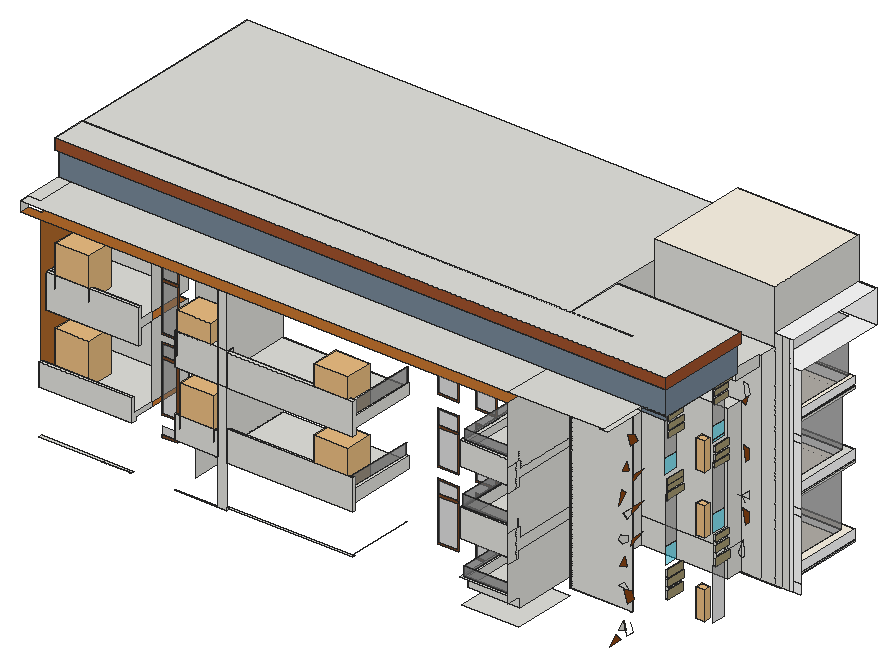
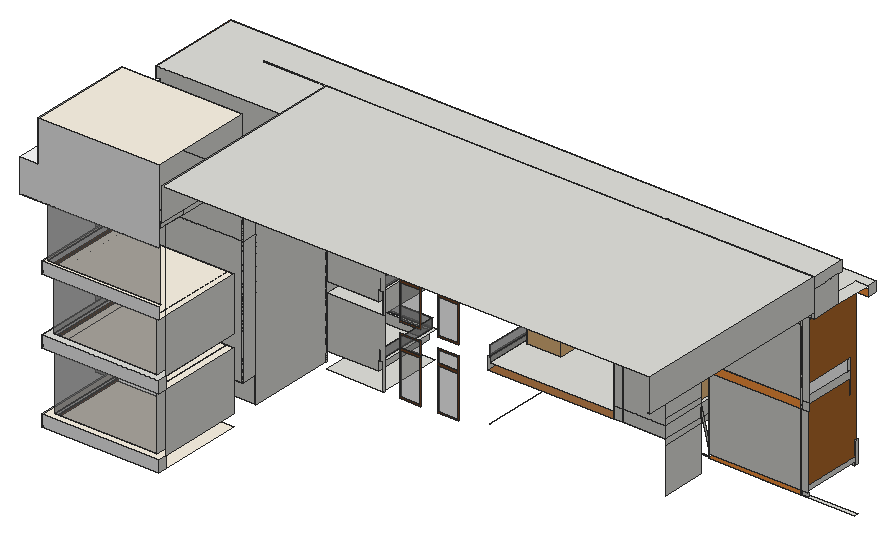
# SketchUp Ruby script. Lengths in inches.
U = 1.inch
M = Sketchup.active_model
def pt(a) = Geom::Point3d.new(a.map { |v| v * U })
def face(e, loops, mat)
  f = e.add_face(loops[0].map { |a| pt(a) })
  loops[1..].each { |l| e.add_face(l.map { |a| pt(a) }).erase! }
  f.material = f.back_material = mat if mat
  f
end
# faces: each face lists its corners as indices into pts; further lists are holes
def faces(e, pts, list, mat = nil) = list.each { |f| face(e, (f[0].is_a?(Array) ? f : [f]).map { |l| l.map { |i| pts[i] } }, mat) }
# xy, xz, yz: faces in a plane at the given z, y or x. An outline is a flat list of corners, or four numbers for a rectangle; further outlines are holes
def ring(l) = l.size == 4 ? [[l[0], l[1]], [l[2], l[1]], [l[2], l[3]], [l[0], l[3]]] : l.each_slice(2).to_a
def flat(e, list, mat, &to3) = list.each { |f| face(e, (f[0].is_a?(Array) ? f : [f]).map { |l| ring(l).map { |u, v| to3.(u, v) } }, mat) }
def xy(e, z, list, mat = nil) = flat(e, list, mat) { |x, y| [x, y, z] }
def xz(e, y, list, mat = nil) = flat(e, list, mat) { |x, z| [x, y, z] }
def yz(e, x, list, mat = nil) = flat(e, list, mat) { |y, z| [x, y, z] }
def lines(e, pts, list) = list.each { |a, b| e.add_line(pt(pts[a]), pt(pts[b])) }
# prism: a flat outline (further loops are holes) pulled along v
def prism(e, loops, v, mat = nil)
  f = face(e, loops, mat); d = Geom::Vector3d.new(v.map { |x| x * U })
  f.pushpull(f.normal.samedirection?(d) ? d.length : -d.length)
end
def box(e, o, s, mat = nil) = prism(e, [[o, [o[0] + s[0], o[1], o[2]], [o[0] + s[0], o[1] + s[1], o[2]], [o[0], o[1] + s[1], o[2]]]], [0, 0, s[2]], mat)
def at(x, y, z, deg = 0) = Geom::Transformation.translation(pt([x, y, z])) * Geom::Transformation.rotation(ORIGIN, Z_AXIS, deg.degrees)
def axes(o, x, y, z) = Geom::Transformation.new([*x, 0, *y, 0, *z, 0, *pt(o).to_a, 1])
def part(name) = M.definitions.add(name)
# library, detail: a bought-in or finely detailed component or shape, given as its bounding box
def library(name, o, s) = part(name).tap { |d| box(d.entities, o, s) }
def detail(e, o, s) = box(e.add_group.entities, o, s)
def put(e, d, t, mat = nil) = e.add_instance(d, t).tap { |i| i.material = mat if mat }
def group(e, t, mat = nil) = e.add_group.tap { |g| g.transformation = t; g.material = mat if mat }.entities
root = M.entities
M.materials.add("[0030_OldLace]").color = [253, 245, 230]
M.materials.add("[0042_Sienna]").color = [160, 82, 45]
M.materials.add("[0043_SaddleBrown]").color = [139, 69, 19]
M.materials.add("[0110_LightSlateGray]").color = [119, 136, 153]
M.materials.add("[0128_White]").color = [255, 255, 255]
M.materials.add("[Translucent Glass Gray]").color = [128, 128, 128]
M.materials["[Translucent Glass Gray]"].alpha = 0.5
M.materials.add("[Translucent Glass Tinted]").color = [8, 201, 241]
M.materials["[Translucent Glass Tinted]"].alpha = 0.48
M.materials.add("[Wood Bamboo]").color = [177, 105, 43]
M.materials.add("[Wood Floor]").color = [155, 105, 61]
M.materials.add("[Wood Lumber ButtJoined]").color = [164, 152, 112]
M.materials.add("[Wood Veneer 01]").color = [120, 70, 37]
c1 = library("WALL+LIGHT+69",[4.19,4.05,-9.67],[4.61,5.7,18.91])
c2 = library("Plant+(3)",[-15.5,2.64,0],[117.71,96.38,184.75])
xy(root,304.04,[[1381.11,725.91,1632.4375,929.16]],"[0030_OldLace]")
xy(root,305.16,[[1631,725.91,1632.4375,929.16]])
xy(root,306.29,[[1631,725.91,1632.4375,929.16]])
xy(root,307.875,[[1256.11,342.41,1378.67,480.63]])
xy(root,307.92,[[1631,725.91,1632.4375,929.16]])
xy(root,309.05,[[1631,725.91,1632.4375,929.16]])
xy(root,320.91,[[648.14,329.32,760.05,331.76]])
xy(root,321.16,[[356.17,329.32,555.3,336.26]])
xy(root,322.75,[[1378.67,480.63,1512.23,481.99]])
xy(root,326.04,[[760.05,329.32,1031.24,336.23],[1025.87,336.23,1026.95,480.63]])
xy(root,328.75,[[1381.11,725.91,1381.11,929.16,1632.4375,929.16,1632.4375,725.91,1616.3,725.91,1616.3,913.03,1397.24,913.03,1397.24,725.91]],"[0030_OldLace]")
xy(root,344.1875,[[1266.15,344.87,1378.67,480.63]])
xy(root,364.5625,[[1256.11,335.28,1378.67,335.28,1378.67,340.07,1261.86,340.07,1261.86,480.63,1256.11,480.63],[1263.19,341.7,1378.67,341.7,1378.67,344.87,1266.15,344.87,1266.15,480.63,1263.19,480.63]])
xy(root,379.5625,[[1378.67,669.54,1381.11,703.91],[1381.11,669.54,1567.08,703.91]])
xy(root,385.9375,[[1261.86,340.07,1378.67,340.07,1378.67,341.7,1263.19,341.7,1263.19,480.63,1261.86,480.63]])
xy(root,411.86,[[1627.32,427.98,1631.63,468.55]])
xy(root,413.45,[[760.05,329.32,1031.24,333.68]])
xy(root,417.33,[[648.14,329.32,740.81,330.51]])
xy(root,417.38,[[760.05,333.68,1031.24,334.64]])
xy(root,417.48,[[356.17,329.32,356.17,335.25,540.9,335.25,540.9,341.375,555.3,341.375,555.3,329.32]])
xy(root,417.71,[[1625.18,558.89,1628.93,596.95]])
xy(root,425.41,[[341.11,480.02,356.17,480.63]])
xy(root,425.41,[[356.17,335.25,356.17,480.63,555.3,480.63,555.3,341.375,540.9,341.375,540.9,335.25]],"[Wood Bamboo]")
xy(root,429.39,[[1627.32,427.98,1631.63,468.55]])
xy(root,429.57,[[648.14,330.51,740.81,480.63],[760.05,334.64,1031.24,480.63]],"[Wood Floor]")
xy(root,433.35,[[1625.18,558.89,1628.93,596.95]])
xy(root,434.15,[[356.17,335.79,555.3,480.63],[341.11,480.01,356.17,480.63]])
xy(root,435.78,[[1627.32,427.98,1631.63,470.67]])
xy(root,439.59,[[1256.11,335.28,1378.67,341.89]])
xy(root,443.1,[[1625.18,558.89,1628.93,594.7]])
xy(root,444.84,[[760.05,333.68,1024.58,480.63]])
xy(root,450.52,[[1627.32,427.98,1631.63,470.67]])
xy(root,454.4,[[1627.32,427.98,1631.63,467.8]])
xy(root,455.53,[[648.14,333.49,740.81,480.63],[1026.48,333.68,1031.24,480.63],[1256.11,341.89,1378.67,480.63]])
xy(root,456.06,[[1397.24,725.91,1616.3,913.03]])
xy(root,456.48,[[1381.11,725.91,1632.4375,929.16]],"[0030_OldLace]")
xy(root,457.13,[[1625.18,558.89,1628.93,594.7]])
xy(root,458.99,[[1630.3125,725.91,1632.4375,929.16]])
xy(root,460.73,[[1630.3125,725.91,1632.4375,929.16]])
xy(root,462.54,[[1630.3125,725.91,1632.4375,929.16]])
xy(root,464.25,[[1630.3125,725.91,1632.4375,929.16]])
xy(root,464.84,[[1625.18,558.89,1628.93,594.2]])
xy(root,466.46,[[356.17,329.32,555.3,335.79]])
xy(root,467.97,[[648.14,329.32,740.81,333.49]])
xy(root,468.47,[[1627.32,427.98,1631.63,467.8]])
xy(root,476.71,[[1625.18,558.89,1628.93,594.2]])
xy(root,478.58,[[1265.15,344.3125,1378.67,480.63]])
xy(root,478.66,[[760.05,329.32,1031.24,333.68],[1024.58,333.68,1026.48,480.63]])
xy(root,482.34,[[1381.11,725.91,1381.11,929.16,1632.4375,929.16,1632.4375,725.91,1617.91,725.91,1617.91,914.63,1395.63,914.63,1395.63,728.87,1583.5,728.87,1583.5,725.91]])
xy(root,500.08,[[1256.11,335.28,1378.67,335.28,1378.67,339.79,1260.73,339.79,1260.73,480.63,1256.11,480.63],[1261.13,340.29,1378.67,340.29,1378.67,344.3125,1265.15,344.3125,1265.15,480.63,1261.13,480.63]])
xy(root,523.64,[[1260.73,339.79,1378.67,339.79,1378.67,340.29,1261.13,340.29,1261.13,480.63,1260.73,480.63]])
xy(root,558.06,[[648.14,329.32,760.05,347.69],[760.05,329.32,1031.24,337.57]])
xy(root,558.97,[[356.17,347.69,555.3,353.19]])
xy(root,572.25,[[648.14,331.57,740.81,347.69]])
xy(root,572.25,[[760.05,337.57,1031.24,480.63],[648.14,347.69,740.81,480.63]],"[Wood Floor]")
xy(root,578.13,[[1256.11,335.28,1378.67,342.54]])
xy(root,588.63,[[760.05,337.57,1026.8,480.63]])
xy(root,590.28,[[341.11,479.78,356.17,480.63]])
xy(root,590.28,[[356.17,353.19,555.3,480.63]],"[Wood Bamboo]")
xy(root,595.76,[[648.14,331.57,740.81,480.63],[1028.375,337.57,1031.24,480.63],[1256.11,342.54,1378.67,480.63]])
xy(root,597.41,[[1583.5,725.91,1583.5,728.87,1395.63,728.87,1395.63,914.63,1617.91,914.63,1617.91,725.91]])
xy(root,598.78,[[1381.11,725.91,1632.4375,929.16]],"[0030_OldLace]")
xy(root,602.32,[[1630.1875,725.91,1632.4375,929.16]])
xy(root,604.08,[[1630.1875,725.91,1632.4375,929.16]])
xy(root,605.18,[[1629.07,427.98,1631.5,469.55]])
xy(root,605.42,[[1630.3125,725.91,1632.4375,929.16]])
xy(root,606.8,[[1623.49,558.89,1627.24,595.51]])
xy(root,607.68,[[1630.3125,725.91,1632.4375,929.16]])
xy(root,607.98,[[356.17,355.38,555.3,479.76]])
xy(root,611.84,[[1268.92,348.09,1378.67,480.63]])
xy(root,616.24,[[1623.49,558.89,1627.24,595.51]])
xy(root,616.93,[[1629.07,427.98,1631.5,469.55]])
xy(root,620.41,[[1624.9,558.89,1628.78,594.07]])
xy(root,621.03,[[1629.07,427.98,1631.5,468.05]])
xy(root,624.41,[[1625.07,725.91,1625.07,922.47,1381.11,922.47,1381.11,929.16,1632.4375,929.16,1632.4375,725.91]],"[0030_OldLace]")
xy(root,625.94,[[760.05,329.32,1031.24,337.57],[1026.8,337.57,1028.375,480.63]])
xy(root,628.4,[[1256.11,335.28,1378.67,335.28,1378.67,341.58,1262.51,341.58,1262.51,480.63,1256.11,480.63],[1263.04,342.52,1378.67,342.52,1378.67,348.09,1268.92,348.09,1268.92,480.63,1263.04,480.63]])
xy(root,629.13,[[648.14,329.32,760.05,347.69]])
xy(root,630.5,[[1629.07,427.98,1631.5,468.05]])
xy(root,630.91,[[1624.9,558.89,1628.78,594.07]])
xy(root,631.73,[[356.17,347.69,555.3,355.38]])
xy(root,633.43,[[1629.07,427.98,1631.5,467.67]])
xy(root,636.65,[[1624.78,558.89,1628.78,594.34]])
xy(root,643.95,[[1629.07,427.98,1631.5,467.67]])
xy(root,649.25,[[1624.78,558.89,1628.78,594.34]])
xy(root,649.4,[[1262.51,341.58,1263.04,480.63],[1263.04,341.58,1378.67,342.52]])
xy(root,651.9375,[[1378.67,669.54,1567.08,703.91]])
xy(root,723.3125,[[1630.2,427.98,1632.07,468.05]])
xy(root,728.9,[[1624.7,558.89,1626.82,594.34]])
xy(root,735.53,[[1630.2,427.98,1632.07,468.05]])
xy(root,738.98,[[1381.11,922.47,1583.5,929.53]])
xy(root,738.98,[[1625.07,725.91,1678.36,725.91,1678.36,929.53,1583.5,929.53,1583.5,922.47,1625.07,922.47]],"[0128_White]")
xy(root,739.45,[[1630.2,427.98,1632.07,469.17]])
xy(root,740.75,[[1624.7,558.89,1626.82,594.34]])
xy(root,745.11,[[1624.7,558.89,1626.82,593.95]])
xy(root,747.5625,[[740.81,329.32,760.05,480.63]])
xy(root,750.7,[[1630.2,427.98,1632.07,469.17]])
xy(root,751.9375,[[555.3,384.82,648.14,479.76]])
xy(root,752.13,[[328.44,313.35,328.44,334.16,356.17,334.16,356.17,384.82,648.14,384.82,648.14,480.63,1378.67,480.63,1378.67,313.35],[356.17,384.82,648.14,415.98],[356.17,415.98,648.14,479.76]],"[Wood Bamboo]")
xy(root,755.19,[[1624.7,558.89,1626.82,593.95]])
xy(root,757.41,[[1618,606,1635.25,666.21]])
xy(root,757.6,[[1630.2,427.98,1632.07,467.07]])
xy(root,758.84,[[1624.7,558.89,1626.82,606]])
xy(root,764,[[1566.87,325.97,1584.12,415.98]])
xy(root,767.17,[[1624.7,558.89,1626.82,606]])
xy(root,768.01,[[1630.2,427.98,1632.07,467.07]])
xy(root,770.68,[[1621.75,427.98,1636.25,467.07],[1632.37,467.07,1636.25,558.89],[1621.75,558.89,1636.25,594.34]])
xy(root,774.125,[[328.44,313.35,1378.67,313.35,1379.01,415.98,356.17,415.98,356.17,334.16,328.44,334.16],[1378.67,313.35,1584.12,313.35,1584.12,415.98,1379.01,415.98],[328.44,334.16,356.17,415.98],[328.44,479.76,341.11,480.63]])
xy(root,781.4375,[[1378.67,606,1635.25,606,1635.25,666.21,1639.62,666.21,1639.62,703.91,1378.67,703.91]])
xy(root,784.875,[[341.11,479.76,356.17,480.63],[328.44,480.63,334.36,922.03],[334.36,480.63,341.11,863.91],[1378.67,480.63,1381.11,480.63,1381.11,703.91,1380.23,703.91,1380.59,789.03,1380.91,863.91,1380.91,922.03,1378.67,922.03]])
xy(root,808.62,[[1639.62,703.91,1678.36,929.53]],"[0128_White]")
xy(root,831.95,[[328.44,405.29,328.44,415.98,1636.25,415.98,1636.25,606,1644.87,606,1644.87,405.29]],"[Wood Bamboo]")
xy(root,855,[[328.44,405.29,1644.87,405.29,1644.87,606,1378.67,606,1378.67,481.99,1512.23,481.99,1512.23,480.63,648.14,480.63,648.14,479.76,328.44,479.76],[356.17,479.76,648.14,480.63],[328.44,480.63,1378.67,922.03]])
xy(root,897.8125,[[1381.11,703.91,1639.62,929.53]],"[0030_OldLace]")
xz(root,329.32,[[740.81,320.91,760.05,558.06],[555.3,321.06,555.3,321.16,490.96,321.16],[760.05,413.45,1031.24,478.66],[648.14,417.33,740.81,467.97],[356.17,417.48,555.3,466.46],
  [648.14,558.06,740.81,629.13],[740.81,558.06,760.05,629.13],[760.05,558.06,1031.24,625.94],[740.81,629.13,760.05,747.5625]])
xz(root,330.51,[[648.14,417.33,740.81,429.57]])
xz(root,331.57,[[648.14,572.25,740.81,595.76]])
xz(root,333.49,[[648.14,455.53,740.81,467.97]])
xz(root,333.68,[[760.05,413.45,1031.24,417.38],[760.05,444.84,1024.58,478.66],[1026.48,455.53,1031.24,478.66]])
xz(root,334.64,[[760.05,417.38,1031.24,429.57]])
xz(root,335.25,[[356.17,417.48,540.9,425.41]])
xz(root,335.28,[[1256.11,439.59,1378.67,500.08],[1256.11,578.13,1378.67,628.4]])
xz(root,335.79,[[356.17,434.15,555.3,466.46]])
xz(root,337.57,[[760.05,558.06,1031.24,572.25],[760.05,588.63,1026.8,625.94],[1028.375,595.76,1031.24,625.94]])
xz(root,339.79,[[1260.73,500.08,1378.67,523.64]],"[Translucent Glass Gray]")
xz(root,340.07,[[1261.86,364.5625,1378.67,385.9375]],"[Translucent Glass Gray]")
xz(root,340.29,[[1261.13,500.08,1378.67,523.64]],"[Translucent Glass Gray]")
xz(root,341.375,[[540.9,417.48,555.3,425.41]])
xz(root,341.58,[[1262.51,628.4,1263.04,649.4]])
xz(root,341.58,[[1263.04,628.4,1378.67,649.4]],"[Translucent Glass Gray]")
xz(root,341.7,[[1263.19,364.5625,1378.67,385.9375]],"[Translucent Glass Gray]")
xz(root,341.89,[[1256.11,439.59,1378.67,455.53]])
xz(root,342.52,[[1263.04,628.4,1378.67,649.4]],"[Translucent Glass Gray]")
xz(root,342.54,[[1256.11,578.13,1378.67,595.76]])
xz(root,344.3125,[[1265.15,478.58,1378.67,500.08]])
xz(root,344.87,[[1266.15,344.1875,1378.67,364.5625]])
xz(root,347.69,[[648.14,558.06,740.81,572.25],[356.17,558.97,555.3,631.73],[648.14,595.76,736.24,629.13]])
xz(root,348.09,[[1268.92,611.84,1378.67,628.4]])
xz(root,353.19,[[356.17,558.97,555.3,590.28]])
xz(root,355.38,[[356.17,607.98,555.3,631.73]])
xz(root,384.82,[[578.02,378.89,609.9,395.73],[578.83,420.27,609.08,525.18],[578.83,530.5625,609.08,555.125],[578.25,574.6,609.66,673.69],[578.25,679.55,609.66,704.65]],"[Translucent Glass Gray]")
xz(root,384.82,[[575.9,373.61,578.02,378.89],[578.02,373.61,609.9,378.89],[[575.9,417.33,612.02,558.06],[578.83,420.27,609.08,555.125]],[578.83,525.18,609.08,530.5625],[575.9,572.25,612.02,572.25,612.02,707,575.9,707,575.9,679.55,578.25,679.55,578.25,704.65,609.66,704.65,609.66,574.6,578.25,574.6,578.25,673.69,575.9,673.69],
  [575.9,673.69,578.25,679.55],[578.25,673.69,609.66,679.55]],"[Wood Veneer 01]")
xz(root,405.29,[[328.44,831.95,1644.87,855]],"[0042_Sienna]")
xz(root,415.98,[[1584.12,764,1636.25,770.68],[1584.12,770.68,1636.25,774.125],[328.44,774.125,1636.25,831.95]],"[0110_LightSlateGray]")
xz(root,427.98,[[1627.32,429.39,1631.63,435.78],[1627.32,450.52,1631.63,454.4],[1629.07,602.14,1631.5,605.18],[1629.07,616.93,1631.5,618.39],[1629.07,618.39,1631.5,621.03],
  [1629.07,630.5,1631.5,633.43],[1630.2,735.53,1632.07,739.45],[1630.2,739.45,1632.07,750.7],[1630.2,750.7,1632.07,757.6],[1630.2,768.01,1632.07,769.27]])
xz(root,467.07,[[1630.2,757.6,1632.07,768.01],[1632.07,766.85,1632.37,768.01]])
xz(root,467.67,[[1629.07,633.43,1631.5,643.95]])
xz(root,467.8,[[1627.32,454.4,1631.63,468.47]])
xz(root,468.05,[[1629.07,621.03,1631.5,630.5],[1630.2,723.3125,1632.07,735.53]])
xz(root,468.55,[[1627.32,411.86,1631.63,429.39]])
xz(root,469.17,[[1630.2,739.45,1632.07,750.7]])
xz(root,469.55,[[1629.07,605.18,1631.5,616.93]])
xz(root,470.67,[[1627.32,435.78,1631.63,450.52]])
xz(root,479.76,[[341.11,607.98,356.17,774.125],[356.17,607.98,555.3,752.13],[555.3,751.9375,648.14,752.13],[356.17,752.13,555.3,774.125],[555.3,752.13,648.14,774.125],
  [328.44,774.125,341.11,784.875],[341.11,774.125,356.17,784.875],[356.17,774.125,555.3,784.875],[555.3,774.125,648.14,784.875],[328.44,784.875,356.17,831.95],
  [356.17,784.875,648.14,831.95],[328.44,831.95,356.17,855],[356.17,831.95,648.14,855]])
xz(root,480.63,[[1253.63,307.875,1256.11,307.875,1256.11,364.5625,1261.86,364.5625,1261.86,385.9375,1263.19,385.9375,1263.19,364.5625,1266.15,364.5625,1266.15,344.1875,1378.67,344.1875,1378.67,455.53,1253.63,455.53],[1378.67,322.75,1381.11,784.875],[1381.11,322.75,1381.11,784.875,1378.67,784.875,1378.67,855,1512.23,855,1512.23,322.75],[648.14,429.57,740.81,455.53],[740.81,429.57,760.05,455.53],
  [341.11,434.15,356.17,590.28],[356.17,434.15,555.3,590.28],[648.14,455.53,740.81,572.25],[740.81,455.53,760.05,572.25],[1253.63,455.53,1256.11,455.53,1256.11,500.08,1260.73,500.08,1260.73,523.64,1261.13,523.64,1261.13,500.08,1265.15,500.08,1265.15,478.58,1378.67,478.58,1378.67,595.76,1253.63,595.76],
  [648.14,572.25,740.81,595.76],[740.81,572.25,1031.24,572.25,1031.24,595.76,1028.375,595.76,1028.375,625.94,1026.8,625.94,1026.8,588.63,760.05,588.63,760.05,595.76,740.81,595.76],[648.14,595.76,740.81,752.13],[740.81,595.76,760.05,747.5625],[1253.63,595.76,1256.11,595.76,1256.11,628.4,1262.51,628.4,1262.51,649.4,1263.04,649.4,1263.04,628.4,1268.92,628.4,1268.92,611.84,1378.67,611.84,1378.67,752.13,1253.63,752.13],
  [740.81,747.5625,760.05,752.13],[648.14,752.13,1253.63,774.125],[1253.63,752.13,1378.67,774.125],[328.44,774.125,334.36,784.875],[334.36,774.125,341.11,784.875],
  [648.14,774.125,1253.63,784.875],[1253.63,774.125,1378.67,784.875],[328.44,784.875,356.17,835.97],[648.14,784.875,1253.63,835.97],[1253.63,784.875,1378.67,835.97],
  [328.44,835.97,356.17,855],[356.17,835.97,648.14,855],[648.14,835.97,1253.63,855],[1253.63,835.97,1378.67,855]])
xz(root,480.63,[[1177.33,310.2,1218.67,399.71],[1095.58,310.625,1136.18,399.4],[1095.58,405.07,1136.18,431],[1177.33,405.07,1218.67,431.42],[1095.58,458.28,1136.18,531.86],
  [1177.83,458.35,1218.18,531.36],[1177.83,536.64,1218.18,567.52],[1095.58,537.12,1136.18,567.59],[1177.5625,598.3125,1218.44,699.87],[1095.86,598.78,1135.9,699.09],
  [1095.86,702.96,1135.9,731.92],[1177.5625,704.26,1218.44,732.38]],"[Translucent Glass Gray]")
xz(root,480.63,[[[1092.83,307.875,1138.93,433.75],[1095.58,310.625,1136.18,431]],[[1175.01,307.875,1221,433.75],[1177.33,310.2,1218.67,431.42]],[1095.58,399.4,1136.18,405.07],[1177.33,399.71,1218.67,405.07],[[1092.83,455.53,1138.93,570.34],[1095.58,458.28,1136.18,567.59]],
  [[1175.01,455.53,1221,570.34],[1177.83,458.35,1218.18,567.52]],[1177.83,531.36,1218.18,536.64],[1095.58,531.86,1136.18,537.12],[[1092.83,595.76,1138.93,734.94],[1095.86,598.78,1135.9,731.92]],[[1175.01,595.76,1221,734.94],[1177.5625,598.3125,1218.44,732.38]],
  [1095.86,699.09,1135.9,702.96],[1177.5625,699.87,1218.44,704.26]],"[Wood Veneer 01]")
xz(root,481.99,[[1378.67,322.75,1512.23,855]])
xz(root,558.89,[[1625.18,433.35,1628.93,443.1],[1625.18,457.13,1628.93,464.84],[1624.7,728.9,1626.82,730.97],[1624.7,740.75,1626.82,745.11],[1624.7,755.19,1626.82,758.84],
  [1624.7,767.17,1626.82,768.15]])
xz(root,593.95,[[1624.7,745.11,1626.82,755.19]])
xz(root,594.07,[[1624.9,620.41,1628.78,630.91]])
xz(root,594.2,[[1625.18,464.84,1628.93,476.71]])
xz(root,594.7,[[1625.18,443.1,1628.93,457.13]])
xz(root,595.51,[[1623.49,606.8,1627.24,616.24]])
xz(root,596.95,[[1625.18,417.71,1628.93,433.35]])
xz(root,606,[[1624.7,758.84,1626.82,767.17],[1635.25,770.68,1636.25,781.4375],[1378.67,781.4375,1378.67,855,1644.87,855,1644.87,831.95,1636.25,831.95,1636.25,781.4375]])
xz(root,669.54,[[1378.67,322.75,1381.11,379.5625],[1381.11,322.75,1567.08,379.5625],[1378.67,379.5625,1567.08,651.9375]])
xz(root,703.91,[[1567.08,322.75,1567.08,651.9375,1381.11,651.9375,1381.11,781.4375,1611.26,781.4375,1611.26,322.75],[1611.26,322.75,1639.62,781.4375],[1639.62,322.75,1655.44,808.62],[1655.44,322.75,1672.48,808.62],[1378.67,379.5625,1380.23,651.9375],
  [1380.23,379.5625,1381.11,651.9375],[1381.11,379.5625,1567.08,651.9375],[1378.67,651.9375,1380.23,781.4375],[1380.23,651.9375,1381.11,781.4375],[1380.23,781.4375,1381.11,784.875],
  [1381.11,781.4375,1639.62,897.8125]])
xz(root,703.91,[[1672.48,322.75,1678.36,808.62]],"[0128_White]")
xz(root,725.91,[[1381.11,328.75,1397.24,328.75,1397.24,456.06,1583.5,456.06,1583.5,456.48,1381.11,456.48],[1381.11,482.34,1583.5,598.78]])
xz(root,725.91,[[1632.4375,306.29,1678.36,306.29,1678.36,328.75,1632.4375,328.75,1632.4375,309.05,1631,309.05,1631,307.92,1632.4375,307.92],[1616.3,328.75,1678.36,328.75,1678.36,456.48,1583.5,456.48,1583.5,456.06,1616.3,456.06],[1632.4375,456.48,1678.36,456.48,1678.36,472.22,1632.4375,472.22,1632.4375,464.25,1630.3125,464.25,1630.3125,462.54,1632.4375,462.54,1632.4375,460.73,1630.3125,460.73,1630.3125,458.99,1632.4375,458.99],[1632.4375,472.22,1678.36,472.22,1678.36,598.78,1583.5,598.78,1583.5,597.41,1617.91,597.41,1617.91,482.34,1632.4375,482.34],[1632.4375,598.78,1678.36,598.78,1678.36,612.6,1632.4375,612.6,1632.4375,607.68,1630.3125,607.68,1630.3125,605.42,1632.4375,605.42,1632.4375,604.08,1630.1875,604.08,1630.1875,602.32,1632.4375,602.32],
  [1632.4375,612.6,1678.36,612.6,1678.36,738.98,1625.07,738.98,1625.07,624.41,1632.4375,624.41]],"[0128_White]")
xz(root,728.87,[[1395.63,482.34,1583.5,597.41]])
xz(root,913.03,[[1397.24,328.75,1616.3,456.06]],"[Translucent Glass Gray]")
xz(root,914.63,[[1395.63,482.34,1617.91,597.41]],"[Translucent Glass Gray]")
xz(root,922.47,[[1381.11,624.41,1625.07,738.98]],"[Translucent Glass Gray]")
xz(root,929.16,[[1381.11,304.04,1632.4375,304.04,1632.4375,305.16,1631,305.16,1631,306.29,1632.4375,306.29,1632.4375,307.92,1631,307.92,1631,309.05,1632.4375,309.05,1632.4375,328.75,1381.11,328.75],[1381.11,456.48,1632.4375,456.48,1632.4375,458.99,1630.3125,458.99,1630.3125,460.73,1632.4375,460.73,1632.4375,462.54,1630.3125,462.54,1630.3125,464.25,1632.4375,464.25,1632.4375,482.34,1381.11,482.34],[1381.11,598.78,1632.4375,598.78,1632.4375,602.32,1630.1875,602.32,1630.1875,604.08,1632.4375,604.08,1632.4375,605.42,1630.3125,605.42,1630.3125,607.68,1632.4375,607.68,1632.4375,624.41,1381.11,624.41]],"[0128_White]")
xz(root,929.53,[[1381.11,738.98,1678.36,738.98,1678.36,808.62,1639.62,808.62,1639.62,897.8125,1381.11,897.8125]],"[0128_White]")
yz(root,328.44,[[313.35,752.13,334.16,774.125],[415.98,774.125,479.76,831.95],[480.63,784.875,922.03,855],[405.29,831.95,479.76,855]])
yz(root,341.11,[[479.76,774.125,480.63,784.875]])
yz(root,356.17,[[329.32,417.48,334.16,466.46],[334.16,417.48,334.16,466.46,335.79,466.46,335.79,434.15,480.01,434.15,480.02,425.41,335.25,425.41,335.25,417.48],[480.02,425.41,480.01,434.15,480.63,434.15,480.63,425.41],[480.01,434.15,479.78,590.28,480.63,590.28,480.63,434.15],[347.69,558.97,347.69,607.98,479.76,607.98,479.78,590.28,353.19,590.28,353.19,558.97],
  [479.78,590.28,479.76,607.98,479.76,784.875,480.63,784.875,480.63,590.28],[347.69,607.98,355.38,631.73],[479.76,784.875,480.63,855]])
yz(root,356.17,[[347.69,558.97,347.69,631.73,479.76,631.73,479.76,607.98,479.78,590.28,353.19,590.28,353.19,558.97],[355.38,607.98,479.76,631.73]],"[0128_White]")
yz(root,356.17,[[335.79,434.15,335.79,466.46,334.16,466.46,334.16,752.13,479.76,752.13,479.76,631.73,347.69,631.73,347.69,558.97,353.19,558.97,353.19,590.28,479.78,590.28,480.01,434.15]],"[Wood Bamboo]")
yz(root,540.9,[[335.25,417.48,341.375,425.41]])
yz(root,555.3,[[329.32,417.48,341.375,417.48,341.375,425.41,384.82,425.41,384.82,434.15,335.79,434.15,335.79,466.46,329.32,466.46],[384.82,434.15,480.63,590.28],[347.69,558.97,353.19,558.97,353.19,590.28,384.82,590.28,384.82,607.98,355.38,607.98,355.38,631.73,347.69,631.73],[384.82,607.98,479.76,751.9375]])
yz(root,648.14,[[384.82,320.91,480.63,417.33],[329.32,417.33,330.51,429.57],[330.51,417.33,384.82,429.57],[384.82,417.33,480.63,429.57],[329.32,429.57,384.82,455.53],
  [384.82,429.57,480.63,455.53],[329.32,455.53,333.49,467.97],[384.82,455.53,480.63,467.97],[384.82,467.97,480.63,558.06],[329.32,558.06,347.69,572.25],
  [347.69,558.06,384.82,572.25],[384.82,558.06,480.63,572.25],[329.32,572.25,331.57,595.76],[331.57,572.25,384.82,595.76],[384.82,572.25,480.63,595.76],
  [329.32,595.76,347.69,629.13],[384.82,595.76,480.63,629.13],[384.82,629.13,480.63,629.13,480.63,752.13,479.76,752.13,479.76,751.9375,384.82,751.9375],[384.82,751.9375,415.98,752.13],[415.98,751.9375,479.76,752.13],
  [479.76,752.13,480.63,774.125],[479.76,774.125,480.63,784.875],[479.76,784.875,480.63,855]])
yz(root,740.81,[[329.32,417.33,330.51,429.57],[329.32,429.57,329.32,467.97,333.49,467.97,333.49,455.53,333.68,455.53,333.68,429.57],[333.68,429.57,480.63,455.53],[333.49,455.53,333.49,467.97,329.32,467.97,329.32,572.25,480.63,572.25,480.63,455.53],[329.32,572.25,331.57,595.76],
  [331.57,572.25,480.63,595.76],[329.32,595.76,480.63,747.5625]])
yz(root,760.05,[[329.32,320.91,331.76,326.04],[329.32,413.45,333.68,429.57],[333.68,417.38,334.64,429.57],[329.32,429.57,480.63,429.57,480.63,444.84,333.68,444.84,333.68,455.53,329.32,455.53],[333.68,444.84,480.63,444.84,480.63,572.25,347.69,572.25,347.69,558.06,329.32,558.06,329.32,478.66,333.68,478.66],
  [329.32,455.53,333.68,478.66],[329.32,558.06,337.57,558.06,337.57,572.25,347.69,572.25,347.69,588.63,337.57,588.63,337.57,625.94,329.32,625.94],[337.57,558.06,347.69,572.25],[347.69,588.63,480.63,588.63,480.63,747.5625,329.32,747.5625,329.32,629.13,347.69,629.13],[337.57,588.63,347.69,625.94],
  [329.32,625.94,347.69,629.13]])
yz(root,1024.58,[[333.68,444.84,480.63,478.66]],"[Translucent Glass Gray]")
yz(root,1026.48,[[333.68,455.53,480.63,478.66]],"[Translucent Glass Gray]")
yz(root,1026.8,[[337.57,588.63,480.63,625.94]],"[Translucent Glass Gray]")
yz(root,1028.375,[[337.57,595.76,480.63,625.94]],"[Translucent Glass Gray]")
yz(root,1031.24,[[329.32,413.45,329.32,478.66,333.68,478.66,333.68,429.57,334.64,429.57,334.64,417.38,333.68,417.38,333.68,413.45],[333.68,429.57,480.63,455.53],[329.32,558.06,337.57,558.06,337.57,572.25,480.63,572.25,480.63,595.76,337.57,595.76,337.57,625.94,329.32,625.94]])
yz(root,1256.11,[[335.28,439.59,335.28,500.08,480.63,500.08,480.63,455.53,341.89,455.53,341.89,439.59],[335.28,578.13,335.28,628.4,480.63,628.4,480.63,595.76,342.54,595.76,342.54,578.13]])
yz(root,1260.73,[[339.79,500.08,480.63,523.64]],"[Translucent Glass Gray]")
yz(root,1261.13,[[340.29,500.08,480.63,523.64]],"[Translucent Glass Gray]")
yz(root,1261.86,[[340.07,364.5625,480.63,385.9375]],"[Translucent Glass Gray]")
yz(root,1262.51,[[341.58,628.4,480.63,649.4]],"[Translucent Glass Gray]")
yz(root,1263.04,[[342.52,628.4,480.63,649.4]],"[Translucent Glass Gray]")
yz(root,1263.19,[[341.7,364.5625,480.63,385.9375]],"[Translucent Glass Gray]")
yz(root,1265.15,[[344.3125,478.58,480.63,500.08]])
yz(root,1266.15,[[344.87,344.1875,480.63,364.5625]])
yz(root,1268.92,[[348.09,611.84,480.63,628.4]])
yz(root,1378.67,[[480.63,322.75,481.99,784.875],[481.99,322.75,481.99,784.875,606,784.875,606,781.4375,669.54,781.4375,669.54,322.75],[344.87,344.1875,344.87,364.5625,341.7,364.5625,341.7,385.9375,340.07,385.9375,340.07,364.5625,313.35,364.5625,313.35,439.59,341.89,439.59,341.89,455.53,480.63,455.53,480.63,344.1875],[669.54,379.5625,703.91,651.9375],[313.35,439.59,335.28,500.08],
  [335.28,439.59,335.28,500.08,339.79,500.08,339.79,523.64,340.29,523.64,340.29,500.08,344.3125,500.08,344.3125,478.58,480.63,478.58,480.63,455.53,341.89,455.53,341.89,439.59],[344.3125,478.58,344.3125,500.08,340.29,500.08,340.29,523.64,339.79,523.64,339.79,500.08,313.35,500.08,313.35,578.13,342.54,578.13,342.54,595.76,480.63,595.76,480.63,478.58],[313.35,578.13,335.28,628.4],[335.28,578.13,335.28,628.4,341.58,628.4,341.58,649.4,342.52,649.4,342.52,628.4,348.09,628.4,348.09,611.84,480.63,611.84,480.63,595.76,342.54,595.76,342.54,578.13],[348.09,611.84,348.09,628.4,342.52,628.4,342.52,649.4,341.58,649.4,341.58,628.4,313.35,628.4,313.35,752.13,480.63,752.13,480.63,611.84],
  [669.54,651.9375,703.91,781.4375],[480.63,784.875,481.99,855],[481.99,784.875,606,855],[606,784.875,922.03,855]])
yz(root,1380.91,[[863.91,774.125,922.03,784.875]])
yz(root,1381.11,[[909.71,304.04,929.16,328.75],[725.91,328.75,909.71,456.48],[909.71,456.48,929.16,482.34],[725.91,482.34,909.71,598.78]])
yz(root,1395.63,[[728.87,482.34,914.63,597.41]])
yz(root,1397.24,[[725.91,328.75,913.03,456.06]])
yz(root,1512.23,[[480.63,322.75,481.99,855]])
yz(root,1567.08,[[669.54,322.75,703.91,379.5625],[669.54,379.5625,703.91,651.9375]])
yz(root,1583.5,[[725.91,482.34,728.87,597.41]])
yz(root,1587.05,[[325.97,350.6,355.59,350.6,341.37,365.85]],"[0043_SaddleBrown]")
yz(root,1587.12,[[369.37,361.78,362.75,384.03,368.62,362.2],[368.62,362.2,362.75,384.03,350.63,372.33]])
yz(root,1588.7,[[389.48,412.57,384.61,432.23,362.75,446.02,371.74,412.6]],"[0043_SaddleBrown]")
yz(root,1591.85,[[355.59,536.57,367.64,536.57,367.64,547.07,349.31,557.0625,343.4,551.36]])
yz(root,1593.42,[[343.8125,616.1875,361.93,633.66,351.48,643.03]],"[0043_SaddleBrown]")
yz(root,1596.5,[[370.97,721.7,389.48,722.28,382.38,737.5625,362.75,746.45]],"[0043_SaddleBrown]")
yz(root,1616.3,[[725.91,328.75,913.03,456.06]],"[Translucent Glass Gray]")
yz(root,1617.91,[[725.91,482.34,914.63,597.41]],"[Translucent Glass Gray]")
yz(root,1621.75,[[560.74,303.84,592.86,415.97],[433.29,507.25,463.16,609.125],[561.04,514.15,592.04,604.41],[430.16,678.39,463.1,769.33],[560.31,683.14,593.12,768.52]],"[Translucent Glass Gray]")
yz(root,1621.75,[[433.29,471.78,463.16,507.25],[561.04,477.54,592.04,514.15],[430.16,647.23,463.1,678.39],[560.31,651.2,593.25,656.77],[560.31,656.77,593.25,683.14]],"[Translucent Glass Tinted]")
yz(root,1623.49,[[558.89,606.8,595.51,616.24]])
yz(root,1624.7,[[558.89,728.9,594.34,740.75],[558.89,745.11,593.95,755.19],[558.89,758.84,606,767.17]])
yz(root,1624.78,[[558.89,636.65,594.34,649.25]])
yz(root,1624.9,[[558.89,620.41,594.07,630.91]])
yz(root,1625.07,[[725.91,624.41,922.47,738.98]],"[Translucent Glass Gray]")
yz(root,1625.18,[[558.89,417.71,596.95,433.35],[558.89,443.1,594.7,457.13],[558.89,464.84,594.2,476.71]])
yz(root,1626.82,[[558.89,728.9,594.34,740.75],[558.89,745.11,593.95,755.19],[558.89,758.84,606,767.17]],"[Wood Lumber ButtJoined]")
yz(root,1627.24,[[558.89,606.8,595.51,616.24]],"[Wood Lumber ButtJoined]")
yz(root,1627.32,[[427.98,411.86,468.55,429.39],[427.98,435.78,470.67,450.52],[427.98,454.4,467.8,468.47]])
yz(root,1628.78,[[558.89,620.41,594.07,630.91],[558.89,636.65,594.34,649.25]],"[Wood Lumber ButtJoined]")
yz(root,1628.93,[[558.89,417.71,596.95,433.35],[558.89,443.1,594.7,457.13],[558.89,464.84,594.2,476.71]],"[Wood Lumber ButtJoined]")
yz(root,1629.07,[[427.98,605.18,469.55,616.93],[427.98,621.03,468.05,630.5],[427.98,633.43,467.67,643.95]])
yz(root,1630.1875,[[725.91,602.32,929.16,604.08]],"[0043_SaddleBrown]")
yz(root,1630.2,[[427.98,723.3125,468.05,735.53],[427.98,739.45,469.17,750.7],[427.98,757.6,467.07,768.01]])
yz(root,1630.3125,[[725.91,458.99,929.16,460.73],[725.91,462.54,929.16,464.25],[725.91,605.42,929.16,607.68]],"[0043_SaddleBrown]")
yz(root,1631,[[725.91,305.16,929.16,306.29],[725.91,307.92,929.16,309.05]],"[0042_Sienna]")
yz(root,1631.46,[[636.11,464.95,643.74,465.75,643.74,486.89,630.06,500.88],[636.11,586.52,644.54,586.56,645.23,606.99,630.61,620.77],[636.62,695.44,643.21,708.05,625.72,708.01]],"[0043_SaddleBrown]")
yz(root,1631.5,[[427.98,605.18,469.55,616.93],[427.98,621.03,468.05,630.5],[427.98,633.43,467.67,643.95]],"[Wood Lumber ButtJoined]")
yz(root,1631.63,[[427.98,411.86,468.55,429.39],[427.98,435.78,470.67,450.52],[427.98,454.4,467.8,468.47]],"[Wood Lumber ButtJoined]")
yz(root,1632.07,[[427.98,723.3125,468.05,735.53],[427.98,739.45,469.17,750.7],[427.98,757.6,467.07,768.01]],"[Wood Lumber ButtJoined]")
yz(root,1632.4375,[[725.91,304.04,929.16,305.16],[725.91,306.29,929.16,307.92],[725.91,456.48,929.16,458.99],[725.91,460.73,929.16,462.54],[725.91,598.78,929.16,602.32],
  [725.91,604.08,929.16,605.42]])
yz(root,1632.4375,[[725.91,309.05,929.16,328.75],[725.91,464.25,929.16,482.34],[725.91,607.68,929.16,624.41]],"[0128_White]")
yz(root,1635.25,[[606,757.41,666.21,781.4375]])
yz(root,1636.25,[[415.98,770.68,606,831.95]],"[0110_LightSlateGray]")
yz(root,1639.62,[[703.91,808.62,929.53,897.8125]])
yz(root,1644.87,[[405.29,831.95,606,855]],"[0042_Sienna]")
p = [[356.17,480.02,425.41],[356.17,480.01,434.15],[341.11,480.01,434.15],[341.11,480.02,425.41],[648.14,384.82,455.53],[555.3,480.63,455.53],
  [555.3,480.63,443.65],[648.14,384.82,443.65],[1590.2,350.63,496.31],[1590.2,367.14,487.31],[1590.27,362.75,508],[1590.2,383.58,534.58],
  [1590.27,379.36,523.25],[1590.2,411.37,534.58],[1591.77,411.37,596.57],[1591.77,383.58,596.57],[1591.85,379.36,585.23],[356.17,479.78,590.28],
  [356.17,479.76,607.98],[341.11,479.76,607.98],[341.11,479.78,590.28],[1593.35,383.58,658.55],[1593.42,379.36,647.22],[1593.35,411.37,658.55],
  [1595,350.63,682.27],[1594.92,367.14,673.27],[1594.92,362.75,693.97],[1380.23,703.91,781.4375],[1380.23,703.91,774.125],[1380.59,789.03,774.125],
  [1380.59,789.03,784.875],[1380.23,703.91,784.875],[1380.91,863.91,774.125],[1380.91,863.91,784.875],[1624.9,558.89,618.75],[1624.78,558.89,618.75],
  [1381.11,909.71,774.125],[1381.11,909.71,598.78],[1379.01,415.98,774.125],[555.3,329.32,417.33],[555.3,329.32,417.48],[507.83,329.32,417.33],
  [1591.85,357.68,596.47],[1591.85,367.01,580.96],[1591.85,355.44,596.44],[1591.85,365.68,579.42],[1588.62,373.96,441.68],[1588.62,363.2,459.56],
  [1588.62,348.05,459.56],[1588.7,364.6875,445.82],[1587.12,366.93,363.91],[1587.12,362.75,384.03],[1587.12,371.74,350.62],[1587.12,368.62,362.2],
  [1587.05,382.38,371.73],[1587.12,389.48,350.58],[1631.46,635.74,708.05],[1631.46,630.61,744.125],[1631.46,643.74,731.82],[1631.46,648.49,710.68],
  [1631.46,636.62,710.68],[1631.46,634.6,508.33],[1631.46,625.82,526.56],[1631.46,647.24,526.56],[1631.46,647.24,510],[1604.02,647.24,510],
  [1631.46,625.82,404.98],[1631.46,616.06,419.91],[1631.46,630.06,440.09],[1630.01,635.37,404.98]]
faces(root,p,[[0,1,2,3],[4,5,6,7],[17,18,19,20],[27,28,29,30,31],[30,29,32,33]])
faces(root,p,[[8,9,10],[11,12,13],[14,15,16],[21,22,23],[24,25,26]],"[0043_SaddleBrown]")
lines(root,p,[[34,35],[36,37],[38,28],[32,36],[39,40],[39,41],[42,43],[43,16],[15,44],[44,45],[45,16],[46,47],
  [47,48],[48,49],[50,51],[52,53],[54,55],[55,52],[56,57],[57,58],[58,59],[59,60],[61,62],[62,63],
  [63,64],[64,65],[66,67],[67,68],[68,69],[69,66]])
put(root,c1,axes([1663.66,489.04,374.96],[0,3.21,0],[-3.21,0,0],[0,0,3.21]))
put(root,c2,axes([384.34,347.69,440.26],[0.62,0,0],[0,0.62,0],[0,0,0.4774]))
put(root,c2,axes([668.2,329.32,442.57],[0.62,0,0],[0,0.62,0],[0,0,0.4774]))
put(root,c2,axes([955.64,329.32,442.57],[0.62,0,0],[0,0.62,0],[0,0,0.4774]))
put(root,c1,axes([1663.66,489.04,536.34],[0,3.21,0],[-3.21,0,0],[0,0,3.21]))
put(root,c2,axes([955.64,329.32,580.51],[0.62,0,0],[0,0.62,0],[0,0,0.4774]))
put(root,c2,axes([661.14,329.32,580.51],[0.62,0,0],[0,0.62,0],[0,0,0.4774]))
put(root,c2,axes([384.34,347.69,604.63],[0.62,0,0],[0,0.62,0],[0,0,0.4774]))
put(root,c1,axes([1663.66,489.04,662.15],[0,3.21,0],[-3.21,0,0],[0,0,3.21]))
